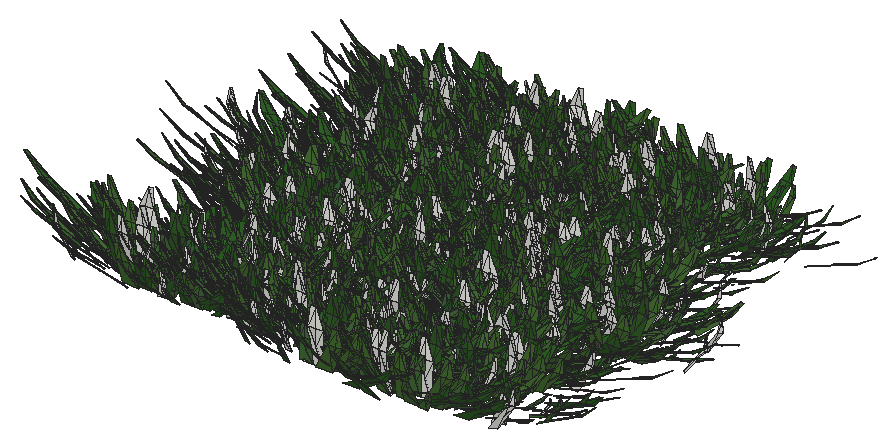
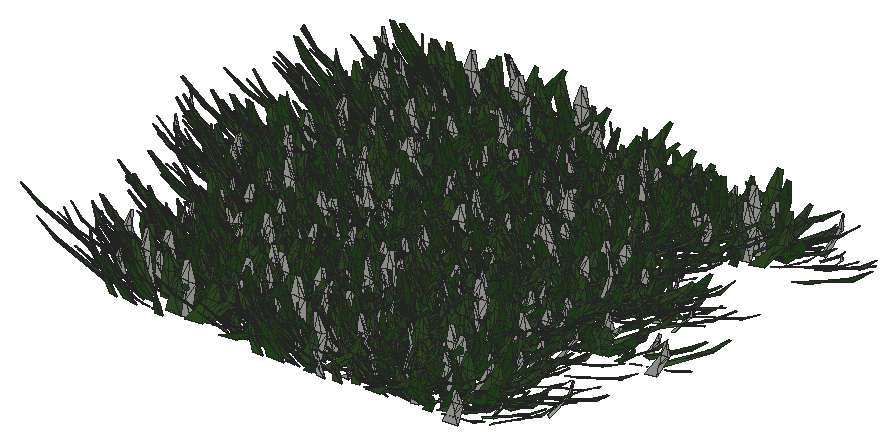
# SketchUp Ruby script. Lengths in inches.
U = 1.inch
M = Sketchup.active_model
def pt(a) = Geom::Point3d.new(a.map { |v| v * U })
def face(e, loops, mat)
  f = e.add_face(loops[0].map { |a| pt(a) })
  loops[1..].each { |l| e.add_face(l.map { |a| pt(a) }).erase! }
  f.material = f.back_material = mat if mat
  f
end
# faces: each face lists its corners as indices into pts; further lists are holes
def faces(e, pts, list, mat = nil) = list.each { |f| face(e, (f[0].is_a?(Array) ? f : [f]).map { |l| l.map { |i| pts[i] } }, mat) }
# xy, xz, yz: faces in a plane at the given z, y or x. An outline is a flat list of corners, or four numbers for a rectangle; further outlines are holes
def ring(l) = l.size == 4 ? [[l[0], l[1]], [l[2], l[1]], [l[2], l[3]], [l[0], l[3]]] : l.each_slice(2).to_a
def flat(e, list, mat, &to3) = list.each { |f| face(e, (f[0].is_a?(Array) ? f : [f]).map { |l| ring(l).map { |u, v| to3.(u, v) } }, mat) }
def xy(e, z, list, mat = nil) = flat(e, list, mat) { |x, y| [x, y, z] }
def xz(e, y, list, mat = nil) = flat(e, list, mat) { |x, z| [x, y, z] }
def yz(e, x, list, mat = nil) = flat(e, list, mat) { |y, z| [x, y, z] }
def lines(e, pts, list) = list.each { |a, b| e.add_line(pt(pts[a]), pt(pts[b])) }
# prism: a flat outline (further loops are holes) pulled along v
def prism(e, loops, v, mat = nil)
  f = face(e, loops, mat); d = Geom::Vector3d.new(v.map { |x| x * U })
  f.pushpull(f.normal.samedirection?(d) ? d.length : -d.length)
end
def box(e, o, s, mat = nil) = prism(e, [[o, [o[0] + s[0], o[1], o[2]], [o[0] + s[0], o[1] + s[1], o[2]], [o[0], o[1] + s[1], o[2]]]], [0, 0, s[2]], mat)
def at(x, y, z, deg = 0) = Geom::Transformation.translation(pt([x, y, z])) * Geom::Transformation.rotation(ORIGIN, Z_AXIS, deg.degrees)
def axes(o, x, y, z) = Geom::Transformation.new([*x, 0, *y, 0, *z, 0, *pt(o).to_a, 1])
def part(name) = M.definitions.add(name)
# library, detail: a bought-in or finely detailed component or shape, given as its bounding box
def library(name, o, s) = part(name).tap { |d| box(d.entities, o, s) }
def detail(e, o, s) = box(e.add_group.entities, o, s)
def put(e, d, t, mat = nil) = e.add_instance(d, t).tap { |i| i.material = mat if mat }
def group(e, t, mat = nil) = e.add_group.tap { |g| g.transformation = t; g.material = mat if mat }.entities
root = M.entities
M.materials.add("Material10").color = [48, 100, 38]
M.materials.add("Material3").color = [68, 110, 58]
M.materials.add("Material4").color = [48, 90, 38]
M.materials.add("Material5").color = [68, 110, 48]
M.materials.add("Material6").color = [48, 90, 48]
M.materials.add("Material7").color = [58, 110, 58]
M.materials.add("Material8").color = [58, 90, 38]
M.materials.add("Material9").color = [68, 100, 58]
c1 = part("grass00")
p = [[-0.6875,0.15,0],[-0.56,0.08,5.52],[-0.04,0.03,2.76],[0.48,-0.02,0],[0.35,-0.02,5.52],[-0.1,-0.14,5.52],
  [-0.12,0.65,8.37],[-0.42,0.65,8.37]]
faces(c1.entities,p,[[0,1,2,3],[3,2,4],[1,5,2],[5,4,2],[1,6,5],[4,5,6],[7,6,1]])
c2 = part("Group16\#1")
put(c2.entities,c1,axes([1.44,-0.61,-0.01],[0.05352,0.12609,0],[-0.10704,0.04543,0.07239],[0.06664,-0.02828,0.11628]),"Material6")
put(c2.entities,c1,axes([0.76,-0.15,-0.01],[0.04676,0.24062,0],[-0.23162,0.04501,0.06642],[0.0652,-0.01267,0.23595]),"Material3")
put(c2.entities,c1,axes([0.79,0.01,-0.01],[-0.00606,0.34651,0],[-0.34381,-0.00602,0.0432],[0.04319,0.00076,0.34386]))
put(c2.entities,c1,axes([1,0.23,-0.01],[-0.07192,0.31144,0],[-0.28722,-0.06632,0.1236],[0.12043,0.02781,0.29478]),"Material5")
put(c2.entities,c1,axes([1.66,0.77,-0.01],[-0.13828,0.29651,0],[-0.21551,-0.1005,0.22471],[0.20365,0.09498,0.23779]),"Material10")
put(c2.entities,c1,axes([0.6875,0.52,-0.01],[-0.18126,0.24051,0],[-0.22746,-0.17142,0.09788],[0.07817,0.05891,0.28481]),"Material5")
put(c2.entities,c1,axes([0.68,0.78,-0.01],[-0.215,0.18688,0],[-0.12385,-0.14248,0.21334],[0.13995,0.16101,0.18878]),"Material3")
put(c2.entities,c1,axes([0.56,1,-0.01],[-0.13756,0.07624,0],[-0.06159,-0.11112,0.0927],[0.04494,0.08108,0.12705]),"Material5")
put(c2.entities,c1,axes([0.2,0.64,-0.01],[-0.23729,0.07254,0],[-0.05711,-0.18681,0.153],[0.04473,0.14632,0.19535]),"Material10")
put(c2.entities,c1,axes([0.0625,0.72,-0.01],[-0.28874,0.02525,0],[-0.02179,-0.24916,0.14647],[0.01276,0.14591,0.25012]),"Material3")
put(c2.entities,c1,axes([-0.08,0.62,-0.01],[-0.34089,-0.04187,0],[0.03255,-0.26504,0.216],[-0.02633,0.21439,0.26703]),"Material10")
put(c2.entities,c1,axes([-0.34,0.98,-0.01],[-0.14314,-0.0493,0],[0.04397,-0.12769,0.06843],[-0.02228,0.0647,0.13505]),"Material10")
put(c2.entities,c1,axes([-0.87,1.45,-0.01],[-0.23488,-0.14114,0],[0.13761,-0.22901,0.06087],[-0.03135,0.05217,0.26717]))
put(c2.entities,c1,axes([-0.72,0.77,-0.01],[-0.14208,-0.13251,0],[0.07209,-0.0773,0.16301],[-0.11118,0.11922,0.1057]),"Material10")
put(c2.entities,c1,axes([-0.62,0.43,-0.01],[-0.14845,-0.21203,0],[0.18654,-0.13061,0.12304],[-0.10079,0.07057,0.22772]),"Material3")
put(c2.entities,c1,axes([-0.68,0.29,-0.01],[-0.13639,-0.32136,0],[0.31723,-0.13464,0.05579],[-0.05136,0.0218,0.34462]),"Material4")
put(c2.entities,c1,axes([-0.64,0.125,-0.01],[-0.0458,-0.23569,0],[0.22124,-0.043,0.08276],[-0.08124,0.01579,0.22538]),"Material7")
put(c2.entities,c1,axes([-1.6,-0.03,-0.01],[0.00576,-0.32897,0],[0.27526,0.00482,0.18018],[-0.18015,-0.00315,0.2753]),"Material5")
put(c2.entities,c1,axes([-1.36,-0.31,-0.01],[0.05718,-0.24765,0],[0.18172,0.04196,0.17267],[-0.16825,-0.03885,0.1865]),"Material10")
put(c2.entities,c1,axes([-1.54,-0.72,-0.01],[0.06537,-0.14017,0],[0.13555,0.06321,0.03939],[-0.0357,-0.01665,0.14956]))
put(c2.entities,c1,axes([-1.19,-0.9,-0.01],[0.09597,-0.12735,0],[0.11214,0.08451,0.07557],[-0.06035,-0.04548,0.14042]),"Material9")
put(c2.entities,c1,axes([-0.47,-0.54,-0.01],[0.11588,-0.10072,0],[0.0618,0.0711,0.12124],[-0.07953,-0.0915,0.0942]))
put(c2.entities,c1,axes([-0.47,-0.84,-0.01],[0.11927,-0.0661,0],[0.06603,0.11913,0.00646],[-0.00313,-0.00565,0.13621]),"Material5")
put(c2.entities,c1,axes([-0.38,-1.24,-0.01],[0.28037,-0.08571,0],[0.0618,0.20215,0.20315],[-0.05939,-0.19428,0.21139]),"Material9")
put(c2.entities,c1,axes([-0.06,-0.66,-0.01],[0.22719,-0.01987,0],[0.01247,0.14255,0.17758],[-0.01547,-0.17691,0.1431]),"Material8")
put(c2.entities,c1,axes([0.11,-0.89,-0.01],[0.14882,0.01828,0],[-0.01058,0.08611,0.12229],[0.01491,-0.12138,0.08676]),"Material6")
put(c2.entities,c1,axes([0.25,-0.72,-0.01],[0.20481,0.07053,0],[-0.06206,0.18022,0.10291],[0.03351,-0.0973,0.1906]),"Material6")
put(c2.entities,c1,axes([0.85,-1.42,-0.01],[0.16481,0.09904,0],[-0.09472,0.15762,0.05616],[0.02893,-0.04814,0.18389]),"Material5")
put(c2.entities,c1,axes([1.01,-1.09,-0.01],[0.21858,0.20385,0],[-0.17495,0.1876,0.15339],[0.10462,-0.11218,0.25652]),"Material10")
put(c2.entities,c1,axes([1.01,-0.71,-0.01],[0.08733,0.12473,0],[-0.06445,0.04512,0.13037],[0.1068,-0.07477,0.07867]),"Material6")
c3 = part("Group15\#1")
put(c3.entities,c2,at(0,0,0))
c4 = part("3darcstudiotree_grass00\#1")
put(c4.entities,c3,at(0,0,0))
put(root,c4,axes([91.85,5.93,7.6],[-0.36246,1.18288,0],[-4.29439,-0.08224,-0.03234],[-0.22764,-0.00436,1.90052]))
put(root,c4,axes([91.51,27.89,7.6],[4.24178,0.73433,0],[-2.3441,0.84628,-0.05103],[-0.19051,0.06878,1.6877]))
put(root,c4,axes([91.94,6.51,7.6],[4.6373,-0.30696,0],[1.13066,1.06758,-0.03329],[0.04185,0.03952,1.35616]))
put(root,c4,axes([92.92,8.9,7.6],[-3.30831,0.84443,0],[-3.70005,-0.906,-0.0181],[-0.07733,-0.01894,1.93624]))
put(root,c4,axes([93.6875,19.36,7.6],[1.24763,-0.92182,0],[4.38061,0.37056,-0.02846],[0.12558,0.01062,1.34635]))
put(root,c4,axes([94.21,20.6,7.6],[1.57584,-0.93457,0],[3.47629,0.36635,-0.03331],[0.19752,0.02082,1.51731]))
put(root,c4,axes([94.22,35.59,7.6],[-2.4775,0.7659,0],[-2.94091,-0.59457,-0.00747],[-0.03328,-0.00673,1.35493]))
put(root,c4,axes([94.36,39.15,7.6],[0.67051,0.95222,0],[-4.84197,0.21309,-0.06022],[-0.34411,0.01514,1.78296]))
put(root,c4,axes([94.38,21.52,7.6],[2.1541,0.73783,0],[-3.48209,0.63537,-0.05552],[-0.23217,0.04236,1.39481]))
put(root,c4,axes([96.5,42.04,7.6],[-1.49369,-1.06151,0],[3.72951,-0.32799,-0.03242],[0.16562,-0.01457,1.33794]))
put(root,c4,axes([97.8125,5.22,7.6],[-4.2486,-0.47023,0],[1.56425,-0.88333,-0.0129],[0.02854,-0.01611,1.31952]))
put(root,c4,axes([96.75,32.15,7.6],[-3.0514,0.75193,0],[-3.33727,-0.84644,-0.00446],[-0.01526,-0.00387,1.44777]))
put(root,c4,axes([97.79,23.125,7.6],[-4.92331,0.15002,0],[-0.48598,-0.99677,-0.03065],[-0.02921,-0.05991,1.97713]))
put(root,c4,axes([98.34,39.9,7.6],[-1.91157,-1.00019,0],[4.33506,-0.51782,-0.00689],[0.03608,-0.00431,1.74288]))
put(root,c4,axes([98.28,36.79,7.6],[-3.45228,-0.31834,0],[1.71903,-1.16515,-0.02933],[0.05627,-0.03814,1.72129]))
put(root,c4,axes([96.89,42.86,7.6],[4.75785,0.13927,0],[-0.57992,1.23828,-0.02723],[-0.01633,0.03486,1.60719]))
put(root,c4,axes([97.31,8.375,7.6],[4.24363,-0.133,0],[0.6088,1.21409,-0.03701],[0.03003,0.05988,1.99511]))
put(root,c4,axes([97.04,27.2,7.6],[4.38323,0.5518,0],[-2.13593,1.06042,-0.03278],[-0.09357,0.04645,1.8841]))
put(root,c4,axes([98.49,22.33,7.6],[1.80526,-0.93773,0],[4.63497,0.55769,-0.06017],[0.29336,0.0353,1.73941]))
put(root,c4,axes([98.33,15.72,7.6],[2.55214,-0.79924,0],[2.90871,0.58051,-0.01018],[0.05177,0.01033,1.51436]))
put(root,c4,axes([97.5,34.14,7.6],[3.99552,0.1688,0],[-0.66851,0.98901,-0.04218],[-0.052,0.07693,1.85529]))
put(root,c4,axes([99.125,12.78,7.6],[-1.20745,-0.91696,0],[4.5972,-0.37835,-0.05688],[0.32578,-0.02681,1.82396]))
put(root,c4,axes([97.43,19.38,7.6],[4.60083,0.27128,0],[-0.99888,1.0588,-0.02883],[-0.04481,0.04749,1.84132]))
put(root,c4,axes([98.52,11.68,7.6],[3.15828,-0.63994,0],[3.01444,0.92981,-0.02341],[0.07838,0.02418,1.59067]))
put(root,c4,axes([99.69,28.09,7.6],[-3.6011,-0.51295,0],[1.91228,-0.83905,-0.01205],[0.03293,-0.01445,1.33255]))
put(root,c4,axes([99.8125,14.51,7.6],[-3.34758,-0.57583,0],[2.35115,-0.85428,-0.02104],[0.0798,-0.02899,1.73448]))
put(root,c4,axes([99.83,35.48,7.6],[-2.89247,-0.63047,0],[2.79907,-0.8026,-0.03875],[0.16322,-0.0468,1.70607]))
put(root,c4,axes([99.02,17.53,7.6],[2.73531,-0.60508,0],[3.15346,0.89096,-0.04815],[0.2108,0.05956,1.9649]))
put(root,c4,axes([98.76,38.43,7.6],[3.9102,0.44615,0],[-1.54008,0.84362,-0.03533],[-0.11802,0.06465,1.86502]))
put(root,c4,axes([99.68,25.33,7.6],[4.11404,0.2026,0],[-0.94809,1.20329,-0.03192],[-0.02927,0.03715,1.45488]))
put(root,c4,axes([100.07,30.85,7.6],[-0.49166,1.00113,0],[-4.41418,-0.13549,-0.03564],[-0.21762,-0.00668,1.71014]))
put(root,c4,axes([99.68,9.44,7.6],[4.50169,0.36178,0],[-1.23301,0.95889,-0.00634],[-0.01342,0.01044,1.74238]))
put(root,c4,axes([100.65,20.37,7.6],[3.54844,-0.68412,0],[2.53941,0.82322,-0.00737],[0.02478,0.00803,1.42978]))
put(root,c4,axes([99.93,6.5625,7.6],[0.51658,1.03873,0],[-3.86244,0.12005,-0.00588],[-0.03275,0.00102,1.36568]))
put(root,c4,axes([99.84,29.96,7.6],[2.79958,0.75017,0],[-3.79275,0.88464,-0.03325],[-0.11995,0.02798,1.59934]))
put(root,c4,axes([102.36,41.9375,7.6],[-3.89596,-0.25813,0],[1.01122,-0.9539,-0.01321],[0.02668,-0.02516,1.9444]))
put(root,c4,axes([102.68,19.57,7.6],[-1.738,-0.84913,0],[4.25665,-0.54453,-0.02541],[0.1,-0.01279,1.32108]))
put(root,c4,axes([102.47,31.52,7.6],[0.41155,-0.92389,0],[4.43873,0.12358,-0.00391],[0.01942,0.00054,1.39627]))
put(root,c4,axes([102.24,27.14,7.6],[0.3191,-1.2505,0],[4.37865,0.06983,-0.05413],[0.27394,0.00437,1.39055]))
put(root,c4,axes([102.45,17.05,7.6],[0.66073,-1.27721,0],[5.08368,0.16437,-0.05291],[0.21846,0.00706,1.33374]))
put(root,c4,axes([102.72,11.91,7.6],[-4.56571,-0.14579,0],[0.54682,-1.07027,-0.0157],[0.01423,-0.02784,1.92971]))
put(root,c4,axes([102.8,40.64,7.6],[0.35405,-1.11937,0],[4.05484,0.08016,-0.00365],[0.02209,0.00044,1.54435]))
put(root,c4,axes([102.86,25.18,7.6],[2.95951,-0.93197,0],[4.0202,0.79789,-0.06314],[0.20058,0.03981,1.30132]))
put(root,c4,axes([103.04,10.16,7.6],[-3.85049,0.40649,0],[-1.93296,-1.14436,-0.01449],[-0.02989,-0.0177,1.64714]))
put(root,c4,axes([104.43,43.35,7.6],[-2.15911,-0.91358,0],[4.38085,-0.64709,-0.05519],[0.27113,-0.04005,1.81465]))
put(root,c4,axes([102.39,20.67,7.6],[2.25416,0.91391,0],[-3.32067,0.5119,-0.00763],[-0.0422,0.0065,1.58363]))
put(root,c4,axes([102.84,29.53,7.6],[4.35171,-0.00299,0],[0.0127,1.15651,-0.02008],[0.00031,0.02806,1.61638]))
put(root,c4,axes([102.97,13.55,7.6],[0.76881,0.99481,0],[-3.92404,0.18954,-0.03785],[-0.21203,0.01024,1.42505]))
put(root,c4,axes([104.79,38.35,7.6],[-3.65156,-0.16407,0],[0.77449,-1.07733,-0.01818],[0.01589,-0.02211,1.35222]))
put(root,c4,axes([105.15,15.97,7.6],[-4.40837,-0.63137,0],[2.29025,-0.99943,-0.04075],[0.1094,-0.04774,1.55523]))
put(root,c4,axes([103.12,28.51,7.6],[4.60532,0.48375,0],[-1.62275,0.96554,-0.00848],[-0.02401,0.01429,1.91304]))
put(root,c4,axes([103.35,14.71,7.6],[4.22855,0.37749,0],[-1.56983,1.09905,-0.00059],[-0.00119,0.00083,1.74794]))
put(root,c4,axes([104.84,34.13,7.6],[2.56038,-0.8827,0],[3.78234,0.6857,-0.00976],[0.05125,0.00929,1.89325]))
put(root,c4,axes([105.2,35.45,7.6],[-0.92872,-0.91526,0],[4.23097,-0.26832,-0.05601],[0.35873,-0.02275,1.80254]))
put(root,c4,axes([105.22,24.09,7.6],[2.77364,-0.77685,0],[3.77594,0.8426,-0.02458],[0.10362,0.02312,1.78746]))
put(root,c4,axes([106.3,32.9,7.6],[-4.1547,-0.33584,0],[1.51583,-1.17203,-0.04655],[0.07348,-0.05682,1.58019]))
put(root,c4,axes([104.91,8.22,7.6],[3.93015,-0.3044,0],[1.10624,0.89267,-0.04073],[0.07417,0.05985,1.43775]))
put(root,c4,axes([104.95,7.06,7.6],[1.67946,0.90749,0],[-4.52669,0.52358,-0.03574],[-0.19906,0.02302,1.91331]))
put(root,c4,axes([105.44,37.4,7.6],[4.66183,0.56246,0],[-1.8815,0.97465,-0.05424],[-0.11893,0.06161,1.36476]))
put(root,c4,axes([106.7,21.68,7.6],[1.39071,-1.04081,0],[3.42496,0.28602,-0.03453],[0.25559,0.02134,1.76116]))
put(root,c4,axes([106.76,5.86,7.6],[0.96858,0.89112,0],[-3.74023,0.25408,-0.02204],[-0.16423,0.01116,1.87051]))
put(root,c4,axes([108.49,15.81,7.6],[-4.69188,-0.0249,0],[0.0963,-1.13384,-0.04949],[0.00708,-0.08333,1.9102]))
put(root,c4,axes([109.5625,36.24,7.6],[-1.9675,-0.8496,0],[3.8564,-0.55817,-0.02105],[0.1271,-0.0184,1.94345]))
put(root,c4,axes([108.67,34.25,7.6],[-3.4865,0.64506,0],[-2.72844,-0.92168,-0.01624],[-0.06139,-0.02074,1.82169]))
put(root,c4,axes([109.16,20.04,7.6],[2.44226,-0.75549,0],[3.06681,0.61963,-0.01488],[0.06384,0.0129,1.35946]))
put(root,c4,axes([110.03,32.61,7.6],[-2.44027,-0.95657,0],[3.80591,-0.60682,-0.04256],[0.19819,-0.0316,1.55835]))
put(root,c4,axes([108.69,40.58,7.6],[3.65585,-0.02969,0],[0.16476,1.26817,-0.05593],[0.00918,0.07069,1.60461]))
put(root,c4,axes([110.16,38.41,7.6],[0.86009,-1.01814,0],[4.02529,0.21253,-0.00249],[0.01488,0.00079,1.57305]))
put(root,c4,axes([109.43,43.35,7.6],[-3.80246,0.84843,0],[-3.3004,-0.92448,-0.01139],[-0.04326,-0.01212,1.76647]))
put(root,c4,axes([110.6875,42.16,7.6],[-0.68955,-0.89341,0],[4.9756,-0.24002,-0.02161],[0.13108,-0.00632,1.95654]))
put(root,c4,axes([110.42,12.83,7.6],[1.44071,-0.87984,0],[4.07175,0.41671,-0.00546],[0.02449,0.00251,1.33158]))
put(root,c4,axes([109.05,29.9,7.6],[1.00747,0.90236,0],[-3.56805,0.24898,-0.02635],[-0.15857,0.01106,1.4463]))
put(root,c4,axes([109.53,37.14,7.6],[-2.23722,1.02937,0],[-4.10468,-0.55756,-0.0267],[-0.10588,-0.01438,1.31753]))
put(root,c4,axes([110.78,4.15,7.6],[1.23489,-1.20152,0],[4.58168,0.29431,-0.01129],[0.06903,0.00443,1.86628]))
put(root,c4,axes([109.08,28.28,7.6],[4.08208,0.66427,0],[-2.13929,0.82165,-0.02904],[-0.11461,0.04402,1.7729]))
put(root,c4,axes([109.88,26.27,7.6],[3.71734,-0.40813,0],[1.8446,1.05006,-0.00525],[0.01214,0.00691,1.64886]))
put(root,c4,axes([110.05,30.78,7.6],[3.61412,-0.47878,0],[2.26101,1.06672,-0.00115],[0.00254,0.0012,1.42878]))
put(root,c4,axes([109.49,17.96,7.6],[3.34943,0.40768,0],[-2.23658,1.14845,-0.05845],[-0.12336,0.06334,1.53958]))
put(root,c4,axes([111.32,11.27,7.6],[-4.90262,0.38062,0],[-1.21174,-0.97549,-0.03919],[-0.07726,-0.06219,1.69748]))
put(root,c4,axes([110.08,23.73,7.6],[4.40316,-0.08214,0],[0.30096,1.00833,-0.02534],[0.0118,0.03954,1.58232]))
put(root,c4,axes([110.6875,7.39,7.6],[3.91548,-0.26914,0],[1.03869,0.94445,-0.03828],[0.06514,0.05923,1.57185]))
put(root,c4,axes([110.51,25.66,7.6],[4.05806,0.27476,0],[-1.0531,0.97211,-0.0432],[-0.06805,0.06282,1.51727]))
put(root,c4,axes([111.33,8.72,7.6],[-2.36017,0.90935,0],[-3.92025,-0.63593,-0.05659],[-0.22736,-0.03688,1.39892]))
put(root,c4,axes([112.51,22.17,7.6],[3.07578,-0.55136,0],[2.5802,0.89961,-0.04704],[0.16898,0.05892,1.70604]))
put(root,c4,axes([111.62,5.42,7.6],[3.3125,0.68522,0],[-3.11487,0.94112,-0.00662],[-0.02265,0.00684,1.63949]))
put(root,c4,axes([112.52,18.8,7.6],[4.72223,0.15279,0],[-0.65977,1.27445,-0.04718],[-0.02776,0.05361,1.4726]))
put(root,c4,axes([112.8,10.01,7.6],[0.9264,1.21479,0],[-3.78487,0.1804,-0.03349],[-0.21957,0.01047,1.60736]))
put(root,c4,axes([114.44,10.53,7.6],[-3.0009,-0.56917,0],[2.28303,-0.75232,-0.01586],[0.06179,-0.02036,1.52204]))
put(root,c4,axes([112.77,14.66,7.6],[4.12875,0.54518,0],[-1.92192,0.90969,-0.05015],[-0.16609,0.07861,1.82381]))
put(root,c4,axes([114.45,24.15,7.6],[3.49538,-0.78655,0],[2.6672,0.74081,-0.02235],[0.11606,0.03224,1.93391]))
put(root,c4,axes([115.14,28.66,7.6],[2.53666,-1.01382,0],[4.04089,0.63191,-0.01393],[0.05733,0.00897,1.44657]))
put(root,c4,axes([115.2,42.13,7.6],[-4.33002,0.49068,0],[-1.86161,-1.02674,-0.00714],[-0.01364,-0.00752,1.30481]))
put(root,c4,axes([115.5,19.29,7.6],[2.06526,-1.11645,0],[4.68232,0.54135,-0.01],[0.05596,0.00647,1.98774]))
put(root,c4,axes([114.64,17.93,7.6],[-2.02693,0.82712,0],[-3.18296,-0.48751,-0.01687],[-0.08389,-0.01285,1.36079]))
put(root,c4,axes([116,5.0625,7.6],[1.53918,-1.14465,0],[4.66766,0.39228,-0.02131],[0.11149,0.00937,1.69918]))
put(root,c4,axes([115.3,14.83,7.6],[2.64191,-0.97906,0],[3.33396,0.56227,-0.04469],[0.26935,0.04543,1.8275]))
put(root,c4,axes([116.51,26.88,7.6],[-3.19126,-0.77471,0],[2.91337,-0.75007,-0.03796],[0.16003,-0.0412,1.58175]))
put(root,c4,axes([114.8,37.03,7.6],[-0.05785,0.90621,0],[-4.99492,-0.01993,-0.04794],[-0.2528,-0.00101,1.64652]))
put(root,c4,axes([115.99,29.11,7.6],[1.75969,-1.05403,0],[3.90588,0.40755,-0.05171],[0.2964,0.03093,1.64301]))
put(root,c4,axes([117.24,39.08,7.6],[-1.78532,-1.2019,0],[4.51139,-0.41883,-0.00006],[0.00036,-0.00003,1.81412]))
put(root,c4,axes([115.45,39.96,7.6],[0.51329,0.95207,0],[-4.68245,0.15778,-0.05207],[-0.31247,0.01053,1.7882]))
put(root,c4,axes([117.21,11.12,7.6],[-3.2892,-0.91562,0],[3.69199,-0.82892,-0.05274],[0.25135,-0.05643,1.98669]))
put(root,c4,axes([115.41,7.21,7.6],[1.0775,1.11347,0],[-4.72291,0.28565,-0.01063],[-0.05061,0.00306,1.48723]))
put(root,c4,axes([116.26,35.36,7.6],[4.44444,0.2645,0],[-1.11366,1.16958,-0.06215],[-0.07819,0.08211,1.63292]))
put(root,c4,axes([118.25,30.98,7.6],[-3.61007,-0.50137,0],[2.38008,-1.07109,-0.02959],[0.07743,-0.03484,1.65043]))
put(root,c4,axes([116.51,34.35,7.6],[1.61493,0.96375,0],[-4.19905,0.43976,-0.03717],[-0.19495,0.02042,1.61797]))
put(root,c4,axes([116.52,20.6,7.6],[3.19389,0.68135,0],[-2.76112,0.80894,-0.03219],[-0.14851,0.04351,1.88986]))
put(root,c4,axes([116.3,8,7.6],[2.54006,0.86329,0],[-3.88327,0.71411,-0.02079],[-0.07531,0.01385,1.35493]))
put(root,c4,axes([118.72,32.86,7.6],[-4.83306,-0.46342,0],[1.78522,-1.16366,-0.02874],[0.04422,-0.02883,1.33872]))
put(root,c4,axes([118.13,25.43,7.6],[-2.9698,0.72084,0],[-3.26499,-0.84071,-0.01854],[-0.07852,-0.02022,1.78092]))
put(root,c4,axes([118.11,16.35,7.6],[4.49031,-0.36697,0],[1.37458,1.05122,-0.04269],[0.09285,0.07101,1.93529]))
put(root,c4,axes([118.78,12.93,7.6],[3.02119,-0.73797,0],[3.34783,0.85662,-0.03867],[0.15719,0.04022,1.7417]))
put(root,c4,axes([118.36,22.3,7.6],[-0.66076,1.04694,0],[-4.20152,-0.16573,-0.0149],[-0.10633,-0.00419,1.9212]))
put(root,c4,axes([120.94,26.52,7.6],[-4.31344,-0.70765,0],[2.03692,-0.77599,-0.04657],[0.20265,-0.0772,1.84036]))
put(root,c4,axes([120.625,5.27,7.6],[1.44261,-1.06055,0],[4.32057,0.36732,-0.01889],[0.12331,0.01048,1.96679]))
put(root,c4,axes([120.52,31.16,7.6],[2.7969,-0.77222,0],[3.1053,0.70294,-0.04299],[0.19432,0.04399,1.59659]))
put(root,c4,axes([121.5,4.35,7.6],[-3.32225,-0.97797,0],[3.38352,-0.71838,-0.05304],[0.28473,-0.06045,1.95407]))
put(root,c4,axes([121.44,32.82,7.6],[-4.68241,-0.00671,0],[0.02158,-0.94079,-0.00073],[0.00003,-0.00117,1.50826]))
put(root,c4,axes([120.74,34.18,7.6],[-2.30847,0.97502,0],[-3.8485,-0.56948,-0.03668],[-0.22363,-0.03309,1.98009]))
put(root,c4,axes([121.17,17.01,7.6],[-3.40463,0.90031,0],[-2.90136,-0.68574,-0.02847],[-0.11642,-0.02752,1.40417]))
put(root,c4,axes([121.65,35.44,7.6],[-3.76475,0.39529,0],[-1.59865,-0.95161,-0.01995],[-0.04859,-0.02892,1.62326]))
put(root,c4,axes([120.99,43.47,7.6],[-1.90201,1.02558,0],[-4.52641,-0.52466,-0.04346],[-0.2357,-0.02732,1.86413]))
put(root,c4,axes([121.28,10.32,7.6],[-2.71864,0.85934,0],[-2.93369,-0.58007,-0.01059],[-0.0476,-0.00941,1.33934]))
put(root,c4,axes([122.33,23.89,7.6],[-4.9722,0.10596,0],[-0.33395,-0.9794,-0.04632],[-0.03038,-0.08909,1.89764]))
put(root,c4,axes([120.59,37.67,7.6],[3.97374,0.24333,0],[-1.22585,1.25118,-0.01455],[-0.02127,0.02171,1.97892]))
put(root,c4,axes([123.34,24.58,7.6],[-4.53093,-0.46907,0],[1.45069,-0.87579,-0.00358],[0.00956,-0.00577,1.65637]))
put(root,c4,axes([122.34,29.33,7.6],[-1.34638,0.95238,0],[-3.42274,-0.30242,-0.03966],[-0.22852,-0.02019,1.38647]))
put(root,c4,axes([122.87,21.01,7.6],[-3.83366,0.85497,0],[-2.76672,-0.77537,-0.04505],[-0.16078,-0.04506,1.39266]))
put(root,c4,axes([123.9,27.61,7.6],[-1.48823,-0.96446,0],[4.19205,-0.40429,-0.03571],[0.22835,-0.02202,1.92492]))
put(root,c4,axes([122.37,41.9,7.6],[2.1454,0.98431,0],[-3.66531,0.49931,-0.025],[-0.16769,0.02284,1.99255]))
put(root,c4,axes([124.18,22.07,7.6],[-4.49935,0.03553,0],[-0.13779,-1.09065,-0.03959],[-0.00757,-0.05991,1.65212]))
put(root,c4,axes([123.24,14.89,7.6],[3.94822,-0.31947,0],[1.46453,1.13124,-0.01611],[0.0264,0.02039,1.58139]))
put(root,c4,axes([122.53,15.46,7.6],[3.048,0.98317,0],[-3.94868,0.7651,-0.03267],[-0.16044,0.03109,1.93988]))
put(root,c4,axes([122.71,39.3,7.6],[1.55836,1.05765,0],[-4.59334,0.423,-0.04046],[-0.19369,0.01784,1.56076]))
put(root,c4,axes([122.82,12.49,7.6],[0.02941,0.96921,0],[-5.11425,0.0097,-0.03677],[-0.15931,0.0003,1.38481]))
put(root,c4,axes([124.72,6.79,7.6],[-4.27197,-0.09913,0],[0.4691,-1.26352,-0.06502],[0.02705,-0.07286,1.42798]))
put(root,c4,axes([123.68,18.87,7.6],[-0.64236,0.88776,0],[-3.75703,-0.1699,-0.01415],[-0.08369,-0.00378,1.43376]))
put(root,c4,axes([124.81,11.46,7.6],[1.50582,-1.13859,0],[4.62077,0.38195,-0.04027],[0.21526,0.01779,1.71232]))
put(root,c4,axes([124.89,39.97,7.6],[3.80605,-0.38984,0],[1.42887,0.87189,-0.00746],[0.01834,0.01119,1.52751]))
put(root,c4,axes([124.27,8.01,7.6],[3.10025,0.78829,0],[-3.57532,0.87883,-0.00938],[-0.04176,0.01026,1.95578]))
put(root,c4,axes([127.21,20.38,7.6],[-1.03913,-0.96879,0],[4.9712,-0.33326,-0.04199],[0.22449,-0.01505,1.7807]))
put(root,c4,axes([127.6,24.8125,7.6],[-2.80799,-0.72862,0],[3.20036,-0.77086,-0.03217],[0.13224,-0.03185,1.58546]))
